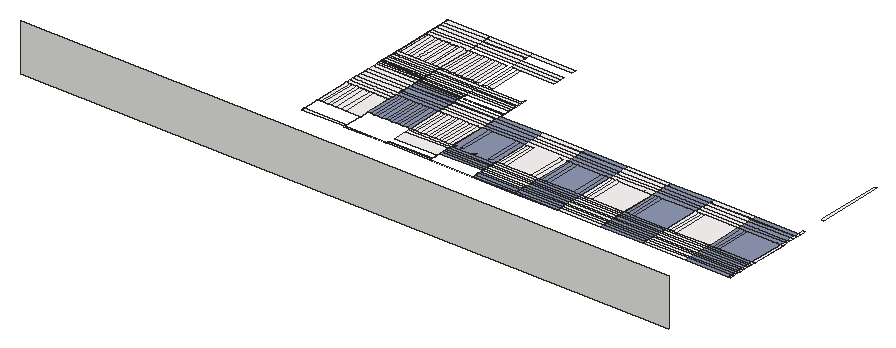
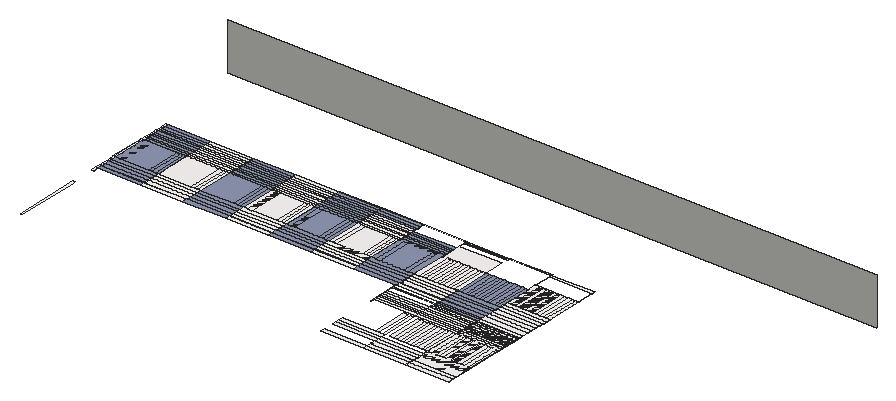
# SketchUp Ruby script. Lengths in inches.
U = 1.inch
M = Sketchup.active_model
def pt(a) = Geom::Point3d.new(a.map { |v| v * U })
def face(e, loops, mat)
  f = e.add_face(loops[0].map { |a| pt(a) })
  loops[1..].each { |l| e.add_face(l.map { |a| pt(a) }).erase! }
  f.material = f.back_material = mat if mat
  f
end
# faces: each face lists its corners as indices into pts; further lists are holes
def faces(e, pts, list, mat = nil) = list.each { |f| face(e, (f[0].is_a?(Array) ? f : [f]).map { |l| l.map { |i| pts[i] } }, mat) }
# xy, xz, yz: faces in a plane at the given z, y or x. An outline is a flat list of corners, or four numbers for a rectangle; further outlines are holes
def ring(l) = l.size == 4 ? [[l[0], l[1]], [l[2], l[1]], [l[2], l[3]], [l[0], l[3]]] : l.each_slice(2).to_a
def flat(e, list, mat, &to3) = list.each { |f| face(e, (f[0].is_a?(Array) ? f : [f]).map { |l| ring(l).map { |u, v| to3.(u, v) } }, mat) }
def xy(e, z, list, mat = nil) = flat(e, list, mat) { |x, y| [x, y, z] }
def xz(e, y, list, mat = nil) = flat(e, list, mat) { |x, z| [x, y, z] }
def yz(e, x, list, mat = nil) = flat(e, list, mat) { |y, z| [x, y, z] }
def lines(e, pts, list) = list.each { |a, b| e.add_line(pt(pts[a]), pt(pts[b])) }
# prism: a flat outline (further loops are holes) pulled along v
def prism(e, loops, v, mat = nil)
  f = face(e, loops, mat); d = Geom::Vector3d.new(v.map { |x| x * U })
  f.pushpull(f.normal.samedirection?(d) ? d.length : -d.length)
end
def box(e, o, s, mat = nil) = prism(e, [[o, [o[0] + s[0], o[1], o[2]], [o[0] + s[0], o[1] + s[1], o[2]], [o[0], o[1] + s[1], o[2]]]], [0, 0, s[2]], mat)
def at(x, y, z, deg = 0) = Geom::Transformation.translation(pt([x, y, z])) * Geom::Transformation.rotation(ORIGIN, Z_AXIS, deg.degrees)
def axes(o, x, y, z) = Geom::Transformation.new([*x, 0, *y, 0, *z, 0, *pt(o).to_a, 1])
def part(name) = M.definitions.add(name)
# library, detail: a bought-in or finely detailed component or shape, given as its bounding box
def library(name, o, s) = part(name).tap { |d| box(d.entities, o, s) }
def detail(e, o, s) = box(e.add_group.entities, o, s)
def put(e, d, t, mat = nil) = e.add_instance(d, t).tap { |i| i.material = mat if mat }
def group(e, t, mat = nil) = e.add_group.tap { |g| g.transformation = t; g.material = mat if mat }.entities
root = M.entities
M.materials.add("Niraj_Shirt").color = [144, 153, 181]
M.materials.add("[0010_Snow]").color = [255, 250, 250]
xy(root,3034.69,[[1092.71,2186.8125,1092.71,2258.65,978.84,2258.65,978.84,2362.02,995.58,2362.02,995.58,2266.64,1005.6,2266.64,1005.6,2362.02,1071.08,2362.02,1071.08,2266.64,1082.11,2266.64,1082.11,2362.02,1092.84,2362.02,1092.84,2186.8125],[1093.15,2186.8125,1207.03,2196],[1207.46,2186.8125,1321.34,2196],[1321.34,2186.8125,1321.34,2266.64,1234.22,2266.64,1234.22,2362.02,1321.46,2362.02,1321.46,2186.8125],[1436.09,2186.8125,1549.96,2196],
  [1549.96,2186.8125,1549.96,2266.64,1462.85,2266.64,1462.85,2362.02,1550.09,2362.02,1550.09,2186.8125],[1664.71,2186.8125,1778.59,2196],[1778.59,2186.8125,1778.59,2266.64,1691.47,2266.64,1691.47,2362.02,1778.71,2362.02,1778.71,2186.8125],[1093.15,2196,1207.03,2205.18],[1207.46,2196,1321.34,2205.18],
  [1436.09,2196,1549.96,2205.18],[1664.71,2196,1778.59,2205.18],[1093.15,2205.18,1207.03,2212.6875],[1207.46,2205.18,1321.34,2212.6875],[1436.09,2205.18,1549.96,2212.6875],
  [1664.71,2205.18,1778.59,2212.6875],[1207.46,2212.6875,1321.34,2220.2],[1436.09,2212.6875,1549.96,2220.2],[1664.71,2212.6875,1778.59,2220.2],[978.84,2220.2,1092.71,2227.98],
  [1207.46,2220.2,1321.34,2227.98],[1436.09,2220.2,1549.96,2227.98],[1664.71,2220.2,1778.59,2227.98],[978.84,2227.98,1092.71,2235.76],[1207.46,2227.98,1321.34,2235.76],
  [1436.09,2227.98,1549.96,2235.76],[1664.71,2227.98,1778.59,2235.76],[978.84,2235.76,1092.71,2243.21],[1207.46,2235.76,1321.34,2243.21],[1436.09,2235.76,1549.96,2243.21],
  [1664.71,2235.76,1778.59,2243.21],[978.84,2243.21,1092.71,2250.66],[1207.46,2243.21,1321.34,2250.66],[1436.09,2243.21,1549.96,2250.66],[1664.71,2243.21,1778.59,2250.66],
  [978.84,2250.66,1092.71,2258.65],[1207.46,2250.66,1321.34,2258.65],[1436.09,2250.66,1549.96,2258.65],[1664.71,2250.66,1778.59,2258.65],[1207.46,2258.65,1321.34,2266.64],
  [1436.09,2258.65,1549.96,2266.64],[1664.71,2258.65,1778.59,2266.64],[750.03,2264.48,758.12,2359.87],[758.12,2264.48,766.76,2359.87],[766.76,2264.48,776.78,2359.87],
  [776.78,2264.48,786.79,2359.87],[786.79,2264.48,796.79,2359.87],[796.79,2264.48,805.45,2359.87],[805.45,2264.48,815,2359.87],[815,2264.48,823.63,2359.87],
  [823.63,2264.48,833.62,2359.87],[833.62,2264.48,842.27,2359.87],[842.27,2264.48,853.3,2359.87],[853.3,2264.48,853.3,2359.87,864.03,2359.87,864.03,2265.36,863.9,2265.36,863.9,2264.48],[995.58,2266.64,1005.6,2362.02],
  [1071.08,2266.64,1082.11,2362.02],[1207.46,2266.64,1215.55,2362.02],[1215.55,2266.64,1224.2,2362.02],[1224.2,2266.64,1234.22,2362.02],[1299.7,2266.64,1310.74,2362.02],
  [1436.09,2266.64,1444.18,2362.02],[1444.18,2266.64,1452.83,2362.02],[1452.83,2266.64,1462.85,2362.02],[1664.71,2266.64,1672.8,2362.02],[1672.8,2266.64,1681.45,2362.02],
  [1681.45,2266.64,1691.47,2362.02],[750.03,2359.87,864.03,2372.72],[978.84,2362.02,1092.84,2374.875],[1207.46,2362.02,1321.46,2374.875],[1436.09,2362.02,1550.09,2374.875],
  [1664.71,2362.02,1778.71,2374.875],[750.03,2372.72,750.03,2382.88,863.9,2382.88,863.9,2373.6,864.03,2373.6,864.03,2372.72],[978.84,2374.875,1092.84,2385.03],[1207.46,2374.875,1321.46,2385.03],[1436.09,2374.875,1550.09,2385.03],
  [1664.71,2374.875,1778.71,2385.03],[750.03,2382.88,750.03,2394.99,864.03,2394.99,864.03,2383.75,863.9,2383.75,863.9,2382.88],[978.84,2385.03,1092.84,2397.15],[1207.46,2385.03,1321.46,2397.15],[1436.09,2385.03,1550.09,2397.15],
  [1664.71,2385.03,1778.71,2397.15],[750.03,2394.99,864.03,2408.0625],[978.84,2397.15,1092.84,2409.08],[1207.46,2397.15,1321.46,2409.08],[1436.09,2397.15,1550.09,2409.08],
  [1664.71,2397.15,1778.71,2409.08],[750.03,2409.08,864.03,2420.72],[978.84,2410.21,1092.84,2422.875],[1207.46,2410.21,1321.46,2422.875],[1436.09,2410.21,1550.09,2422.875],
  [1664.71,2410.21,1778.71,2422.875],[750.03,2420.72,864.03,2426.73],[750.34,2426.73,864.03,2433.26],[978.09,2426.73,978.09,2434.13,864.65,2434.13,864.65,2435.91,978.21,2435.91,978.21,2426.73],[1778.65,2426.73,1778.71,2435.41],
  [864.34,2445.09,864.53,2452.6]],"Niraj_Shirt")
xy(root,3034.69,[[750.03,2184.66,863.9,2186.8125],[978.53,2184.66,1092.84,2186.8125],[1092.84,2184.66,1207.15,2186.8125],[1207.15,2184.66,1321.46,2186.8125],[634.96,2186.8125,635.09,2240.3],
  [635.09,2186.8125,635.4,2193.87],[635.4,2186.8125,749.28,2193.87],[749.28,2186.8125,749.4,2240.3],[749.4,2186.8125,749.59,2193.87],[749.59,2186.8125,749.71,2193.84],
  [749.71,2186.8125,750.03,2193.84],[863.78,2186.8125,863.9,2187.23],[863.9,2186.8125,864.03,2194.72],[864.03,2186.8125,864.21,2192.07],[864.21,2186.8125,864.34,2192.07],
  [864.34,2186.8125,977.9,2192.07],[977.9,2186.8125,977.9,2192.07,864.34,2192.07,864.34,2194.72,978.09,2194.72,978.09,2186.8125],[978.09,2186.8125,978.21,2192.07],[978.21,2186.8125,978.4,2194.72],[978.4,2186.8125,978.53,2194.72],
  [978.53,2186.8125,978.84,2266.64],[1092.84,2186.8125,1093.15,2266.64],[1207.03,2186.8125,1207.03,2266.64,1196.43,2266.64,1196.43,2362.02,1185.39,2362.02,1185.39,2266.64,1119.91,2266.64,1119.91,2362.02,1093.15,2362.02,1093.15,2266.64,1093.03,2266.64,1093.03,2362.02,1093.15,2362.02,1093.15,2374.875,1207.15,2374.875,1207.15,2186.8125],[1207.15,2186.8125,1207.46,2266.64],[1321.46,2186.8125,1321.78,2266.64],
  [1321.78,2186.8125,1435.65,2196],[1435.65,2186.8125,1435.65,2266.64,1348.53,2266.64,1348.53,2362.02,1435.78,2362.02,1435.78,2186.8125],[1435.78,2186.8125,1436.09,2266.64],[1550.09,2186.8125,1550.4,2266.64],[1550.4,2186.8125,1664.28,2196],
  [1664.28,2186.8125,1664.28,2266.64,1577.16,2266.64,1577.16,2362.02,1664.4,2362.02,1664.4,2186.8125],[1664.4,2186.8125,1664.71,2266.64],[1778.71,2186.8125,1779.03,2266.64],[1779.03,2186.8125,1784.73,2196],[978.09,2192.07,978.09,2211.41,864.34,2211.41,864.34,2360.74,872.3,2360.74,872.3,2265.36,967.49,2265.36,967.49,2360.74,978.09,2360.74,978.09,2373.6,978.21,2373.6,978.21,2257.37,978.4,2257.37,978.4,2203.9,978.21,2203.9,978.21,2192.07],
  [1321.78,2196,1435.65,2205.18],[1550.4,2196,1664.28,2205.18],[1779.03,2196,1784.73,2205.18],[978.09,2203.9,978.21,2265.36],[1321.78,2205.18,1435.65,2212.6875],
  [1550.4,2205.18,1664.28,2212.6875],[1779.03,2205.18,1784.73,2212.6875],[1093.15,2212.6875,1207.03,2220.2],[1321.78,2212.6875,1435.65,2220.2],[1550.4,2212.6875,1664.28,2220.2],
  [1779.03,2212.6875,1784.73,2220.2],[1093.15,2220.2,1207.03,2227.98],[1321.78,2220.2,1435.65,2227.98],[1550.4,2220.2,1664.28,2227.98],[1779.03,2220.2,1784.73,2227.98],
  [1093.15,2227.98,1207.03,2235.76],[1321.78,2227.98,1435.65,2235.76],[1550.4,2227.98,1664.28,2235.76],[1779.03,2227.98,1784.73,2235.76],[1093.15,2235.76,1207.03,2243.21],
  [1321.78,2235.76,1435.65,2243.21],[1550.4,2235.76,1664.28,2243.21],[1779.03,2235.76,1784.73,2243.21],[635.09,2240.3,635.4,2335.69],[635.4,2240.3,643.49,2335.69],
  [643.49,2240.3,652.14,2335.69],[652.14,2240.3,662.16,2335.69],[662.16,2240.3,672.17,2335.69],[672.17,2240.3,682.17,2335.69],[672.17,2240.3,749.4,2335.69],
  [682.17,2240.3,690.82,2335.69],[690.82,2240.3,700.37,2335.69],[700.37,2240.3,709,2335.69],[709,2240.3,719,2335.69],[719,2240.3,727.64,2335.69],
  [727.64,2240.3,738.68,2335.69],[738.68,2240.3,749.4,2335.69],[749.4,2240.3,749.59,2335.69],[864.34,2241.93,978.09,2249.38],[978.4,2241.93,978.53,2249.38],
  [1093.15,2243.21,1207.03,2250.66],[1321.78,2243.21,1435.65,2250.66],[1550.4,2243.21,1664.28,2250.66],[1779.03,2243.21,1784.73,2250.66],[864.34,2249.38,978.09,2257.37],
  [978.4,2249.38,978.53,2257.37],[1093.15,2250.66,1207.03,2258.65],[1321.78,2250.66,1435.65,2258.65],[1550.4,2250.66,1664.28,2258.65],[1779.03,2250.66,1784.73,2258.65],
  [864.34,2257.37,978.09,2265.36],[978.21,2257.37,978.4,2265.36],[978.4,2257.37,978.53,2265.36],[978.84,2258.65,1092.71,2266.64],[1093.15,2258.65,1207.03,2266.64],
  [1321.78,2258.65,1435.65,2266.64],[1550.4,2258.65,1664.28,2266.64],[1779.03,2258.65,1784.73,2266.64],[749.59,2264.48,749.71,2335.69],[749.71,2264.48,750.03,2359.87],
  [864.03,2265.36,864.21,2359.87],[864.21,2265.36,864.34,2359.87],[864.34,2265.36,872.3,2360.74],[872.3,2265.36,880.95,2360.74],[880.95,2265.36,890.97,2360.74],
  [890.97,2265.36,900.98,2360.74],[900.98,2265.36,910.98,2360.74],[910.98,2265.36,919.63,2360.74],[919.63,2265.36,929.18,2360.74],[929.18,2265.36,937.82,2360.74],
  [937.82,2265.36,947.81,2360.74],[947.81,2265.36,956.45,2360.74],[956.45,2265.36,967.49,2360.74],[978.09,2265.36,978.21,2360.74],[978.21,2265.36,978.4,2360.74],
  [978.4,2265.36,978.53,2360.74],[978.53,2266.64,978.71,2362.02],[978.71,2266.64,978.84,2362.02],[1092.84,2266.64,1093.03,2362.02],[1093.15,2266.64,1101.24,2362.02],
  [1101.24,2266.64,1109.89,2362.02],[1109.89,2266.64,1119.91,2362.02],[1185.39,2266.64,1196.43,2362.02],[1207.15,2266.64,1207.34,2362.02],[1207.34,2266.64,1207.46,2362.02],
  [1321.46,2266.64,1321.65,2362.02],[1321.65,2266.64,1321.78,2362.02],[1321.78,2266.64,1329.87,2362.02],[1329.87,2266.64,1338.51,2362.02],[1338.51,2266.64,1348.53,2362.02],
  [1414.02,2266.64,1425.05,2362.02],[1435.78,2266.64,1435.96,2362.02],[1435.96,2266.64,1436.09,2362.02],[1528.33,2266.64,1539.36,2362.02],[1550.09,2266.64,1550.28,2362.02],
  [1550.28,2266.64,1550.4,2362.02],[1550.4,2266.64,1558.49,2362.02],[1558.49,2266.64,1567.14,2362.02],[1567.14,2266.64,1577.16,2362.02],[1642.64,2266.64,1653.68,2362.02],
  [1664.4,2266.64,1664.59,2362.02],[1664.59,2266.64,1664.71,2362.02],[1756.95,2266.64,1767.99,2362.02],[1778.71,2266.64,1778.9,2362.02],[1778.9,2266.64,1779.03,2362.02],
  [1779.03,2266.64,1784.73,2362.02],[1784.73,2266.64,1787.12,2362.02],[635.09,2335.69,635.4,2348.54],[635.4,2335.69,749.4,2348.54],[749.4,2335.69,749.59,2348.54],
  [749.59,2335.69,749.71,2348.54],[635.09,2348.54,635.4,2358.7],[635.4,2348.54,749.4,2358.7],[749.4,2348.54,749.59,2358.7],[749.59,2348.54,749.71,2358.7],
  [635.09,2358.7,635.4,2370.8125],[635.4,2358.7,749.4,2370.8125],[749.4,2358.7,749.59,2370.8125],[749.59,2358.7,749.71,2370.8125],[749.71,2359.87,750.03,2372.72],
  [864.03,2359.87,864.21,2360.74],[864.21,2359.87,864.34,2360.74],[864.03,2360.74,864.21,2372.72],[864.21,2360.74,864.34,2372.72],[864.34,2360.74,978.09,2373.6],
  [978.09,2360.74,978.21,2373.6],[978.21,2360.74,978.4,2373.6],[978.4,2360.74,978.53,2373.6],[978.53,2362.02,978.84,2409.08],[1092.84,2362.02,1093.15,2409.08],
  [1093.15,2362.02,1207.15,2374.875],[1207.15,2362.02,1207.46,2409.08],[1321.46,2362.02,1321.78,2409.08],[1321.78,2362.02,1435.78,2374.875],[1435.78,2362.02,1436.09,2409.08],
  [1550.09,2362.02,1550.4,2409.08],[1550.4,2362.02,1664.4,2374.875],[1664.4,2362.02,1664.71,2409.08],[1779.03,2362.02,1784.73,2374.875],[635.09,2370.8125,635.4,2383.88],
  [635.4,2370.8125,749.4,2383.88],[749.4,2370.8125,749.59,2383.88],[749.59,2370.8125,749.71,2383.88],[749.71,2372.72,750.03,2382.88],[864.03,2372.72,864.21,2373.6],
  [864.21,2372.72,864.34,2373.6],[863.9,2373.6,864.03,2382.88],[864.03,2373.6,864.21,2382.88],[864.21,2373.6,864.34,2382.88],[864.34,2373.6,978.09,2383.75],
  [978.09,2373.6,978.21,2383.75],[978.21,2373.6,978.4,2383.75],[978.4,2373.6,978.53,2383.75],[1093.15,2374.875,1207.15,2385.03],[1321.78,2374.875,1435.78,2385.03],
  [1550.4,2374.875,1664.4,2385.03],[1779.03,2374.875,1784.73,2385.03],[749.71,2382.88,750.03,2394.99],[863.9,2382.88,864.03,2383.75],[864.03,2382.88,864.21,2383.75],
  [864.21,2382.88,864.34,2383.75],[864.03,2383.75,864.21,2394.99],[864.21,2383.75,864.34,2394.99],[864.34,2383.75,978.09,2395.87],[978.09,2383.75,978.21,2395.87],
  [978.21,2383.75,978.4,2395.87],[978.4,2383.75,978.53,2395.87],[635.09,2383.88,635.4,2396.54],[635.4,2383.88,749.4,2396.54],[749.4,2383.88,749.59,2396.54],
  [749.59,2383.88,749.71,2396.54],[1093.15,2385.03,1207.15,2397.15],[1321.78,2385.03,1435.78,2397.15],[1550.4,2385.03,1664.4,2397.15],[1779.03,2385.03,1784.73,2397.15],
  [749.71,2394.99,750.03,2408.0625],[864.03,2394.99,864.21,2395.87],[864.21,2394.99,864.34,2395.87],[864.03,2395.87,864.21,2408.0625],[864.21,2395.87,864.34,2408.0625],
  [864.34,2395.87,978.09,2408.94],[978.09,2395.87,978.21,2408.94],[978.21,2395.87,978.4,2408.94],[978.4,2395.87,978.53,2408.94],[635.09,2396.54,635.4,2409.08],
  [635.4,2396.54,749.4,2409.08],[749.4,2396.54,749.59,2409.08],[749.59,2396.54,749.71,2409.08],[1093.15,2397.15,1207.15,2409.08],[1321.78,2397.15,1435.78,2409.08],
  [1550.4,2397.15,1664.4,2409.08],[1779.03,2397.15,1784.73,2409.08],[749.71,2408.0625,750.03,2409.08],[750.03,2408.0625,864.03,2409.08],[864.03,2408.0625,864.21,2408.94],
  [864.21,2408.0625,864.34,2408.94],[864.03,2408.94,864.21,2409.08],[864.21,2408.94,864.34,2409.08],[864.34,2408.94,978.21,2409.08],[978.21,2408.94,978.4,2409.08],
  [978.4,2408.94,978.53,2409.08],[635.4,2409.08,749.71,2426.73],[749.71,2409.08,750.03,2420.72],[864.03,2409.08,864.21,2409.95],[864.21,2409.08,864.34,2409.95],
  [864.34,2409.08,978.21,2409.95],[978.21,2409.08,978.4,2409.95],[978.4,2409.08,978.53,2409.95],[978.84,2409.08,1092.84,2410.21],[1093.15,2409.08,1207.15,2410.21],
  [1207.46,2409.08,1321.46,2410.21],[1321.78,2409.08,1435.78,2410.21],[1436.09,2409.08,1550.09,2410.21],[1550.4,2409.08,1664.4,2410.21],[1664.71,2409.08,1778.71,2410.21],
  [1779.03,2409.08,1784.73,2410.21],[864.03,2409.95,864.21,2420.72],[864.21,2409.95,864.34,2420.72],[864.34,2409.95,978.21,2421.59],[978.21,2409.95,978.4,2421.59],
  [978.4,2409.95,978.53,2421.59],[1093.15,2410.21,1207.15,2422.875],[1321.78,2410.21,1435.78,2422.875],[1550.4,2410.21,1664.4,2422.875],[1779.03,2410.21,1784.73,2422.875],
  [749.71,2420.72,750.03,2426.73],[864.03,2420.72,864.21,2421.59],[864.21,2420.72,864.34,2421.59],[864.03,2421.59,864.21,2426.73],[1779.03,2422.875,1779.03,2426.73,1779.09,2426.73,1779.09,2435.41,1784.73,2435.41,1784.73,2422.875],
  [635.4,2426.73,635.53,2435.91],[635.53,2426.73,635.84,2435.91],[635.84,2426.73,749.71,2435.91],[749.71,2426.73,749.84,2433.26],[749.84,2426.73,749.9,2433.26],
  [749.9,2426.73,750.03,2428.42],[750.03,2426.73,750.15,2433.26],[750.15,2426.73,750.34,2433.26],[864.03,2426.73,864.21,2427.6],[978.34,2426.73,978.34,2506.55,978.53,2506.55,978.53,2434.13,978.4,2434.13,978.4,2426.73],
  [864.03,2427.6,864.21,2433.26],[749.9,2428.42,750.03,2433.26],[[749.71,2433.26,749.71,2435.91,635.53,2435.91,635.53,2614.79,635.84,2614.79,635.84,2650.13,749.84,2650.13,749.84,2601.94,739.11,2601.94,739.11,2506.55,749.84,2506.55,749.84,2433.26],[652.58,2506.55,672.6,2601.94],[635.84,2483.125,749.71,2498.5625],[635.84,2438.375,749.71,2450.91],[635.84,2467.9,749.71,2475.68],[635.84,2452.6,749.71,2460.12],[682.61,2506.55,691.26,2601.94],[719.43,2506.55,728.08,2601.94],[700.81,2506.55,709.44,2601.94],[635.84,2506.55,643.93,2601.94]],[749.71,2433.26,749.84,2445.09],[749.84,2433.26,749.9,2435.91],
  [749.9,2433.26,750.03,2435.91],[750.03,2433.26,750.15,2435.91],[750.15,2433.26,750.34,2435.91],[750.34,2433.26,864.21,2435.91],[635.4,2435.91,635.53,2445.09],
  [635.53,2435.91,635.84,2445.09],[749.84,2435.91,749.9,2445.09],[749.9,2435.91,750.03,2435.93],[750.03,2435.91,750.15,2438.375],[750.15,2435.91,750.34,2445.09],
  [750.34,2435.91,864.21,2438.375],[749.9,2435.93,750.03,2443.71],[635.84,2438.375,749.71,2445.09],[750.03,2438.375,750.15,2445.09],[750.34,2438.375,864.21,2445.09],
  [749.9,2443.71,750.03,2445.09],[635.4,2445.09,635.53,2506.55],[635.53,2445.09,635.84,2452.6],[635.84,2445.09,749.71,2450.91],[749.71,2445.09,749.84,2506.55],
  [749.84,2445.09,749.9,2452.6],[749.9,2445.09,750.03,2452.6],[750.03,2445.09,750.15,2452.6],[750.15,2445.09,750.34,2452.6],[750.34,2445.09,864.21,2450.91],
  [750.34,2450.91,864.21,2452.6],[635.53,2452.6,635.84,2460.12],[635.84,2452.6,749.71,2460.12],[749.84,2452.6,749.9,2460.12],[749.9,2452.6,750.03,2458.94],
  [750.03,2452.6,750.15,2460.12],[750.15,2452.6,750.34,2460.12],[750.34,2452.6,864.21,2460.12],[864.65,2452.6,978.21,2460.12],[749.9,2458.94,750.03,2460.12],
  [635.53,2460.12,635.84,2467.9],[635.84,2460.12,749.71,2467.9],[749.84,2460.12,749.9,2467.9],[749.9,2460.12,750.03,2466.39],[750.03,2460.12,750.15,2467.9],
  [750.15,2460.12,750.34,2467.9],[750.34,2460.12,864.21,2467.9],[864.65,2460.12,978.21,2467.9],[749.9,2466.39,750.03,2467.9],[635.53,2467.9,635.84,2475.68],
  [635.84,2467.9,749.71,2475.68],[749.84,2467.9,749.9,2475.68],[749.9,2467.9,750.03,2475.68],[750.03,2467.9,750.15,2475.68],[750.15,2467.9,750.34,2475.68],
  [750.34,2467.9,864.21,2475.68],[864.65,2467.9,978.21,2475.68],[635.53,2475.68,635.84,2483.125],[635.84,2475.68,749.71,2483.125],[749.84,2475.68,750.03,2483.125],
  [750.03,2475.68,750.15,2483.125],[750.15,2475.68,750.34,2483.125],[750.34,2475.68,864.21,2483.125],[864.65,2475.68,978.21,2483.125],[635.53,2483.125,635.84,2490.57],
  [635.84,2483.125,749.71,2490.57],[749.84,2483.125,750.03,2490.57],[750.03,2483.125,750.15,2490.57],[750.15,2483.125,750.34,2490.57],[750.34,2483.125,864.21,2490.57],
  [864.65,2483.125,978.21,2490.57],[635.53,2490.57,635.84,2498.5625],[635.84,2490.57,749.71,2498.5625],[749.84,2490.57,750.03,2498.5625],[750.03,2490.57,750.15,2498.5625],
  [750.15,2490.57,750.34,2498.5625],[750.34,2490.57,864.21,2498.5625],[864.65,2490.57,978.21,2498.5625],[635.53,2498.5625,635.84,2506.55],[635.84,2498.5625,749.71,2506.55],
  [749.84,2498.5625,750.03,2506.55],[750.03,2498.5625,750.15,2506.55],[750.15,2498.5625,750.34,2506.55],[1779.09,2498.5625,1779.09,2506.55,1778.78,2506.55,1778.78,2675.33,1784.73,2675.33,1784.73,2498.5625],[635.4,2506.55,635.53,2675.33],
  [635.53,2506.55,635.84,2601.94],[635.84,2506.55,643.93,2601.94],[643.93,2506.55,652.58,2601.94],[652.58,2506.55,662.6,2601.94],[662.6,2506.55,672.6,2601.94],
  [672.6,2506.55,682.61,2601.94],[682.61,2506.55,691.26,2601.94],[691.26,2506.55,700.81,2601.94],[700.81,2506.55,709.44,2601.94],[709.44,2506.55,719.43,2601.94],
  [719.43,2506.55,728.08,2601.94],[728.08,2506.55,739.11,2601.94],[739.11,2506.55,749.84,2601.94],[749.84,2506.55,750.03,2601.94],[750.03,2506.55,750.15,2601.94],
  [750.15,2506.55,750.34,2601.94],[750.34,2506.55,758.43,2601.94],[758.43,2506.55,767.08,2601.94],[767.08,2506.55,777.1,2601.94],[777.1,2506.55,787.1,2601.94],
  [787.1,2506.55,797.11,2601.94],[797.11,2506.55,805.76,2601.94],[805.76,2506.55,815.31,2601.94],[815.31,2506.55,823.94,2601.94],[823.94,2506.55,833.93,2601.94],
  [833.93,2506.55,842.58,2601.94],[842.58,2506.55,853.61,2601.94],[864.65,2506.55,872.43,2601.94],[881.08,2506.55,891.1,2601.94],[635.53,2601.94,635.84,2614.79],
  [635.84,2601.94,749.84,2614.79],[749.84,2601.94,750.03,2614.79],[750.03,2601.94,750.15,2614.79],[750.15,2601.94,750.34,2614.79],[864.65,2601.94,978.34,2614.79],
  [635.53,2614.79,635.84,2624.95],[635.84,2614.79,749.84,2624.95],[749.84,2614.79,750.03,2624.95],[750.03,2614.79,750.15,2624.95],[750.15,2614.79,750.34,2624.95],
  [750.34,2614.79,864.21,2624.95],[864.65,2614.79,978.34,2624.95],[635.53,2624.95,635.84,2637.0625],[635.84,2624.95,749.84,2637.0625],[749.84,2624.95,750.03,2637.0625],
  [750.03,2624.95,750.15,2637.0625],[750.15,2624.95,750.34,2637.0625],[750.34,2624.95,864.21,2637.0625],[864.65,2624.95,978.34,2637.0625],[635.53,2637.0625,635.84,2650.13],
  [635.84,2637.0625,749.84,2650.13],[749.84,2637.0625,750.03,2650.13],[750.03,2637.0625,750.15,2650.13],[750.15,2637.0625,750.34,2650.13],[750.34,2637.0625,864.21,2650.13],
  [635.53,2650.13,635.84,2662.79],[635.84,2650.13,749.84,2662.79],[749.84,2650.13,750.03,2662.79],[750.03,2650.13,750.15,2651.15],[750.15,2650.13,750.34,2651.15],
  [750.34,2650.13,864.21,2651.15],[864.53,2650.13,864.65,2651.15],[750.03,2651.15,750.15,2662.79],[750.15,2651.15,750.34,2662.79],[750.34,2651.15,864.21,2662.79],
  [750.34,2651.15,864.21,2662.79],[635.53,2662.79,635.84,2675.33],[635.84,2662.79,749.84,2675.33],[749.84,2662.79,750.03,2675.33],[750.03,2662.79,750.15,2668.8],
  [750.15,2662.79,750.34,2668.8],[750.34,2662.79,750.34,2668.8,750.46,2668.8,750.46,2675.33,864.21,2675.33,864.21,2662.79],[864.65,2662.79,978.34,2675.33],[750.03,2668.8,750.15,2675.33],[750.15,2668.8,750.34,2675.33],
  [750.34,2668.8,750.46,2675.33]],"[0010_Snow]")
xz(root,1936.0625,[[80.5,3034.69,1819.6,3161.9375]])
